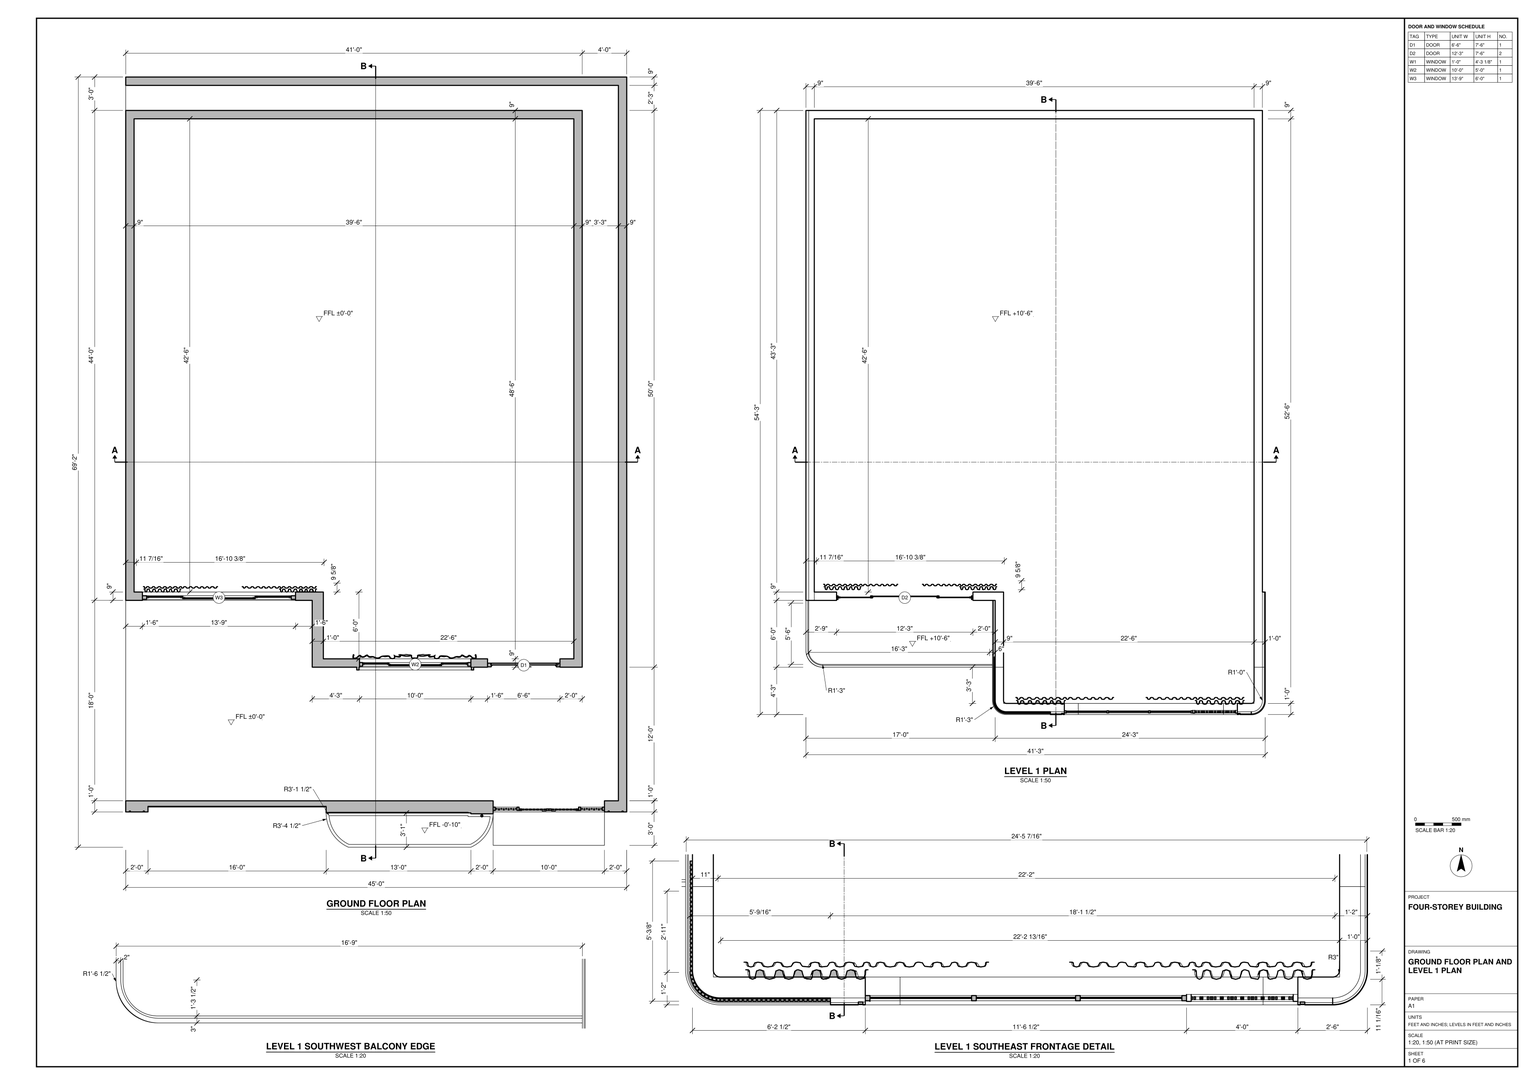
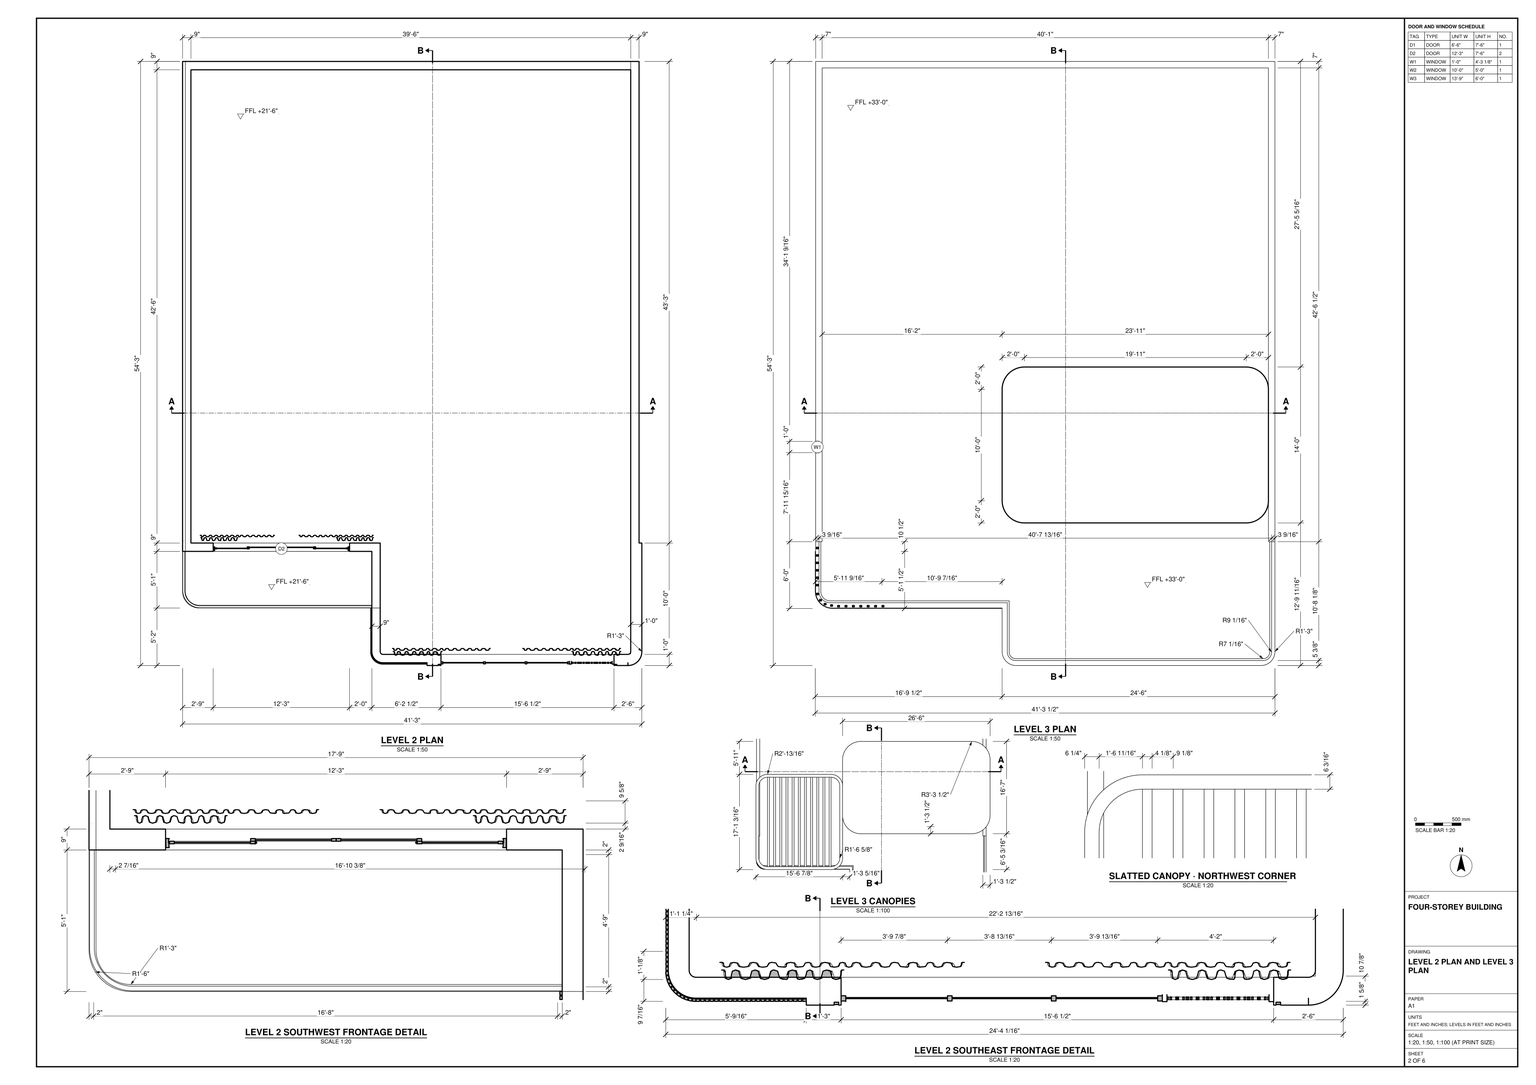
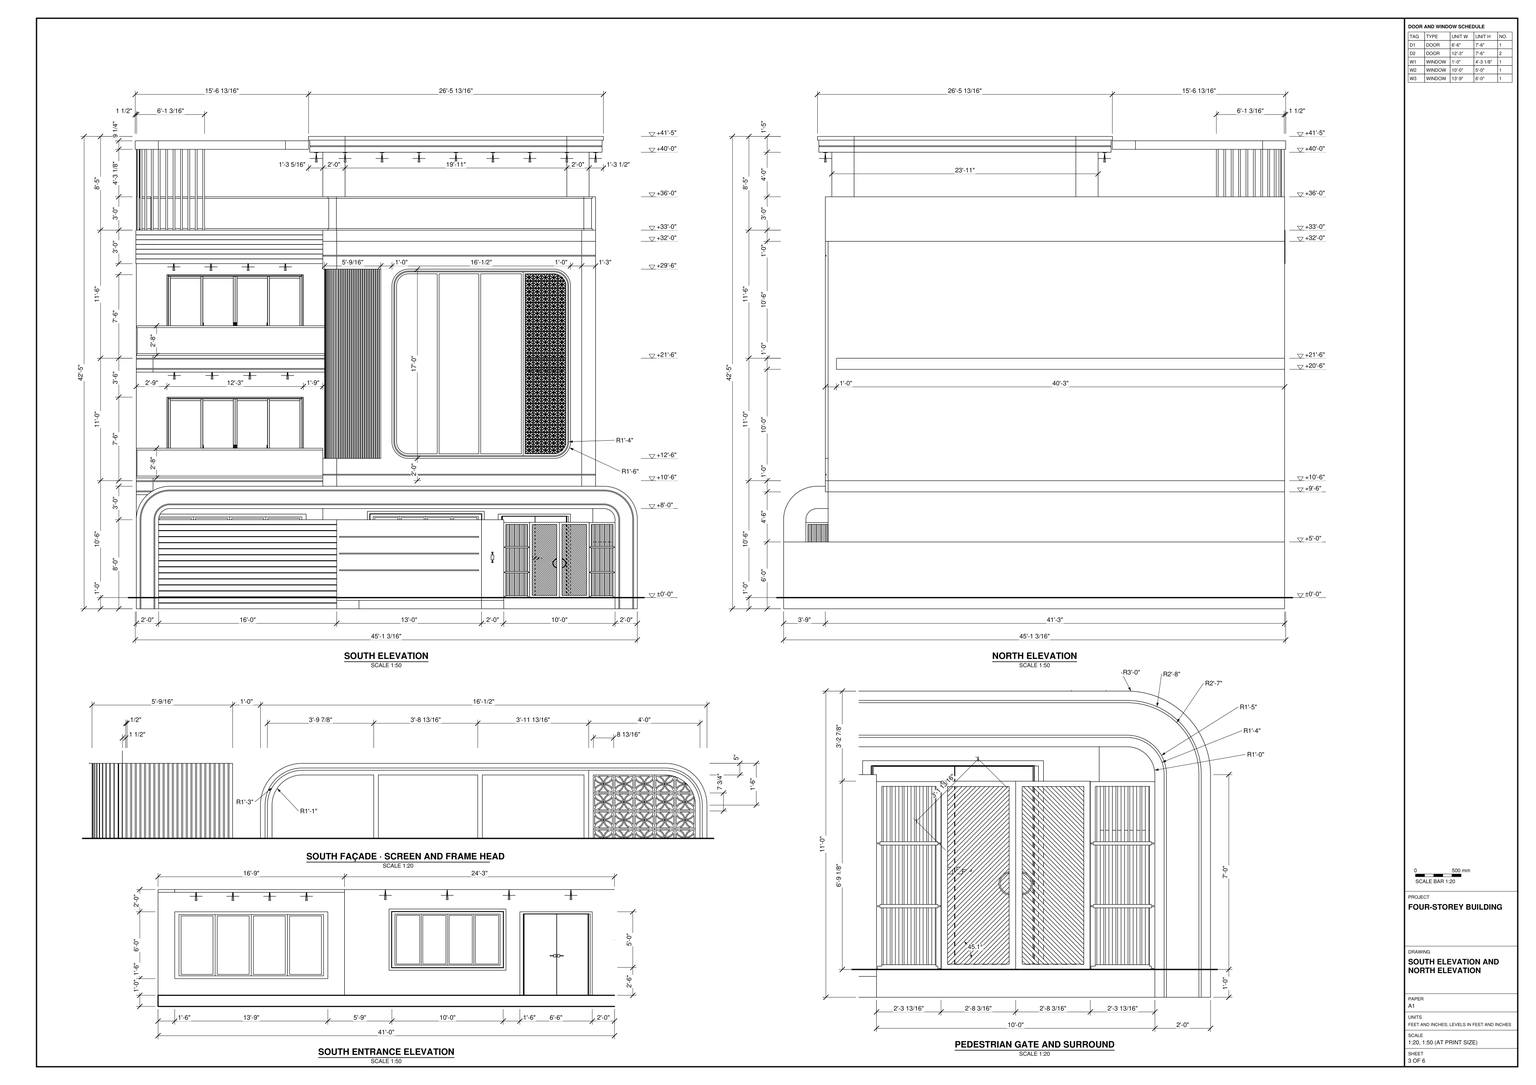
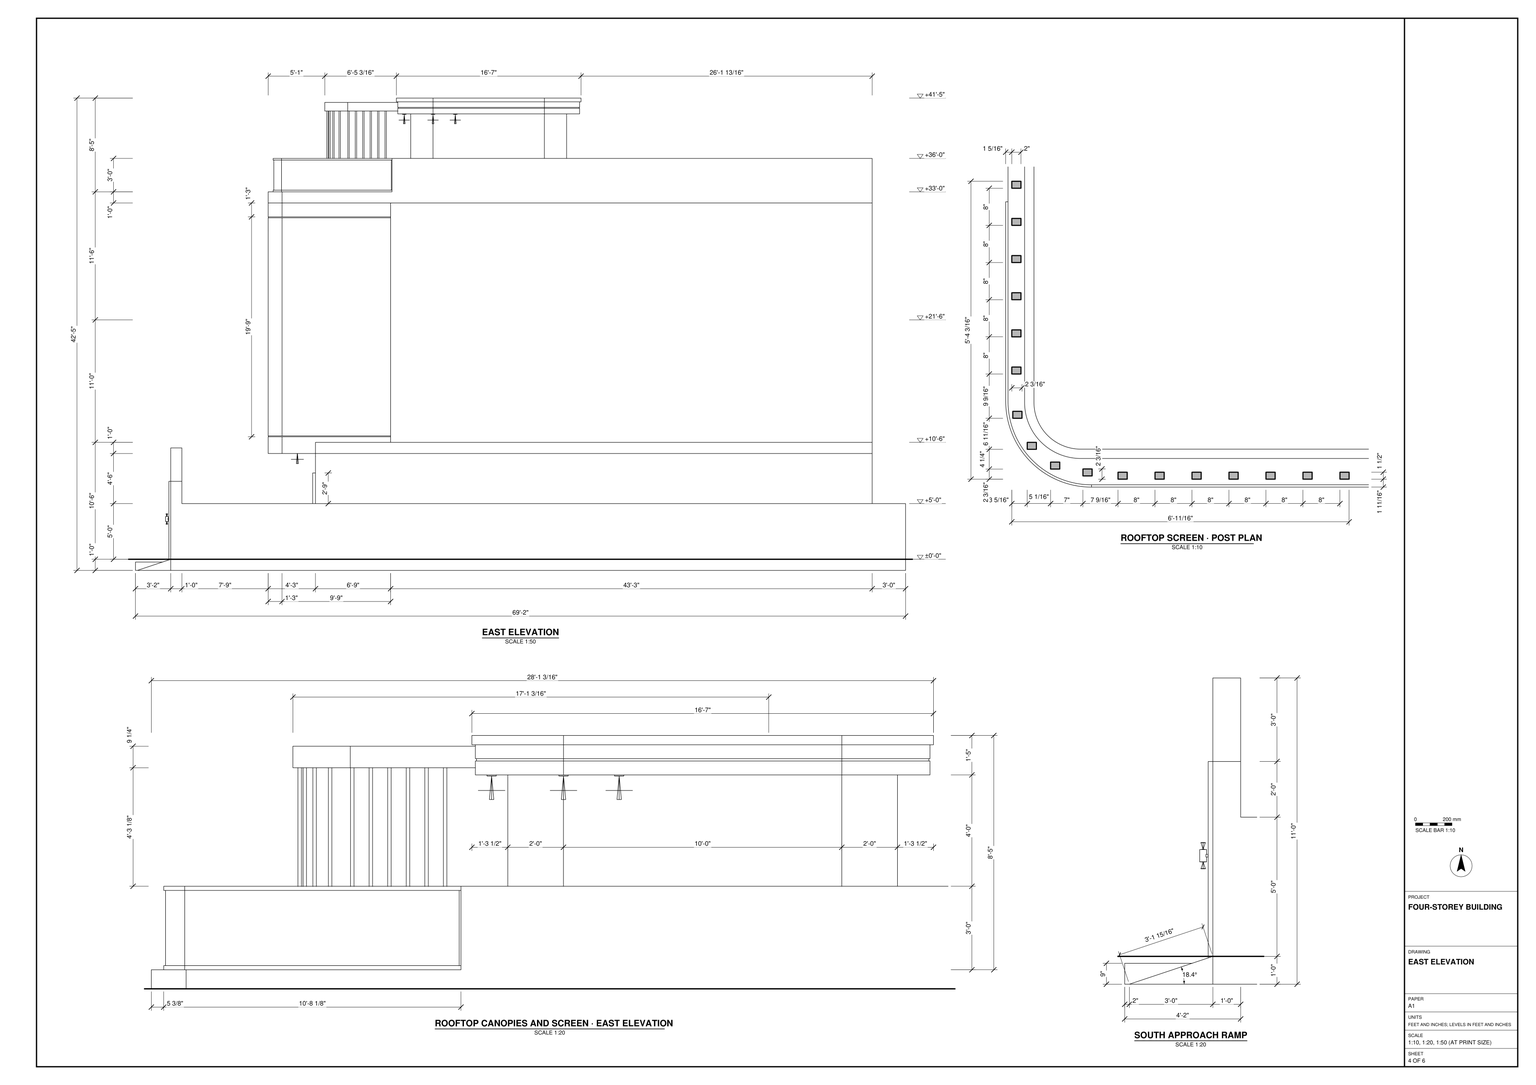
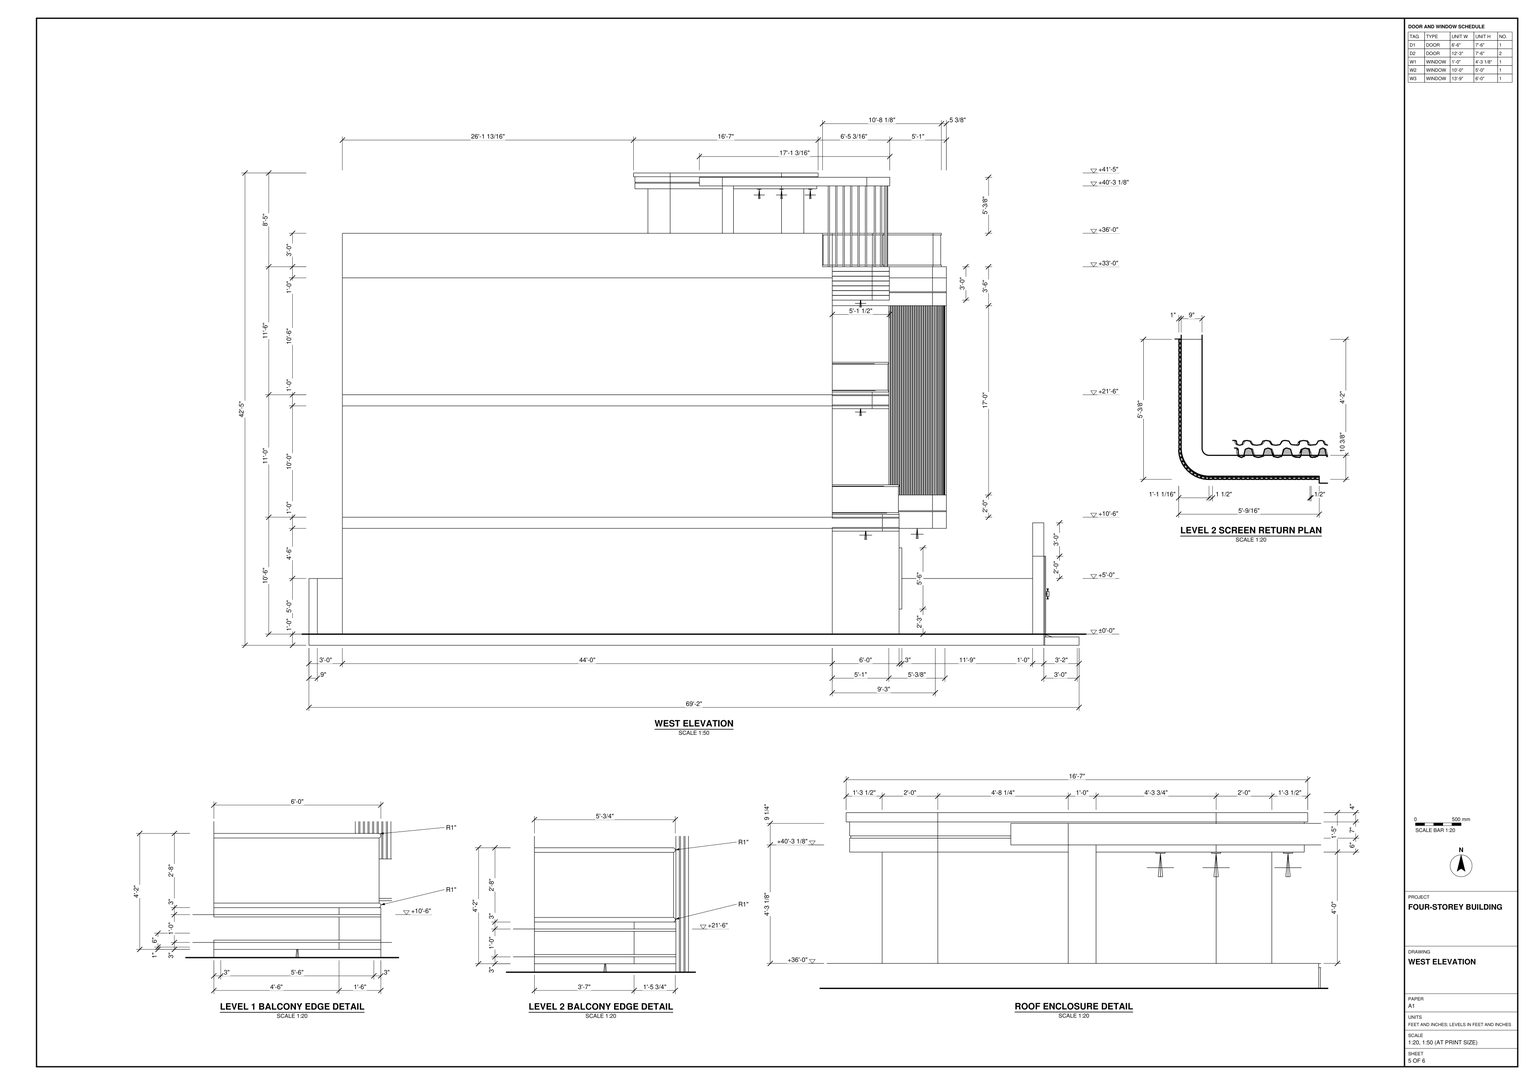
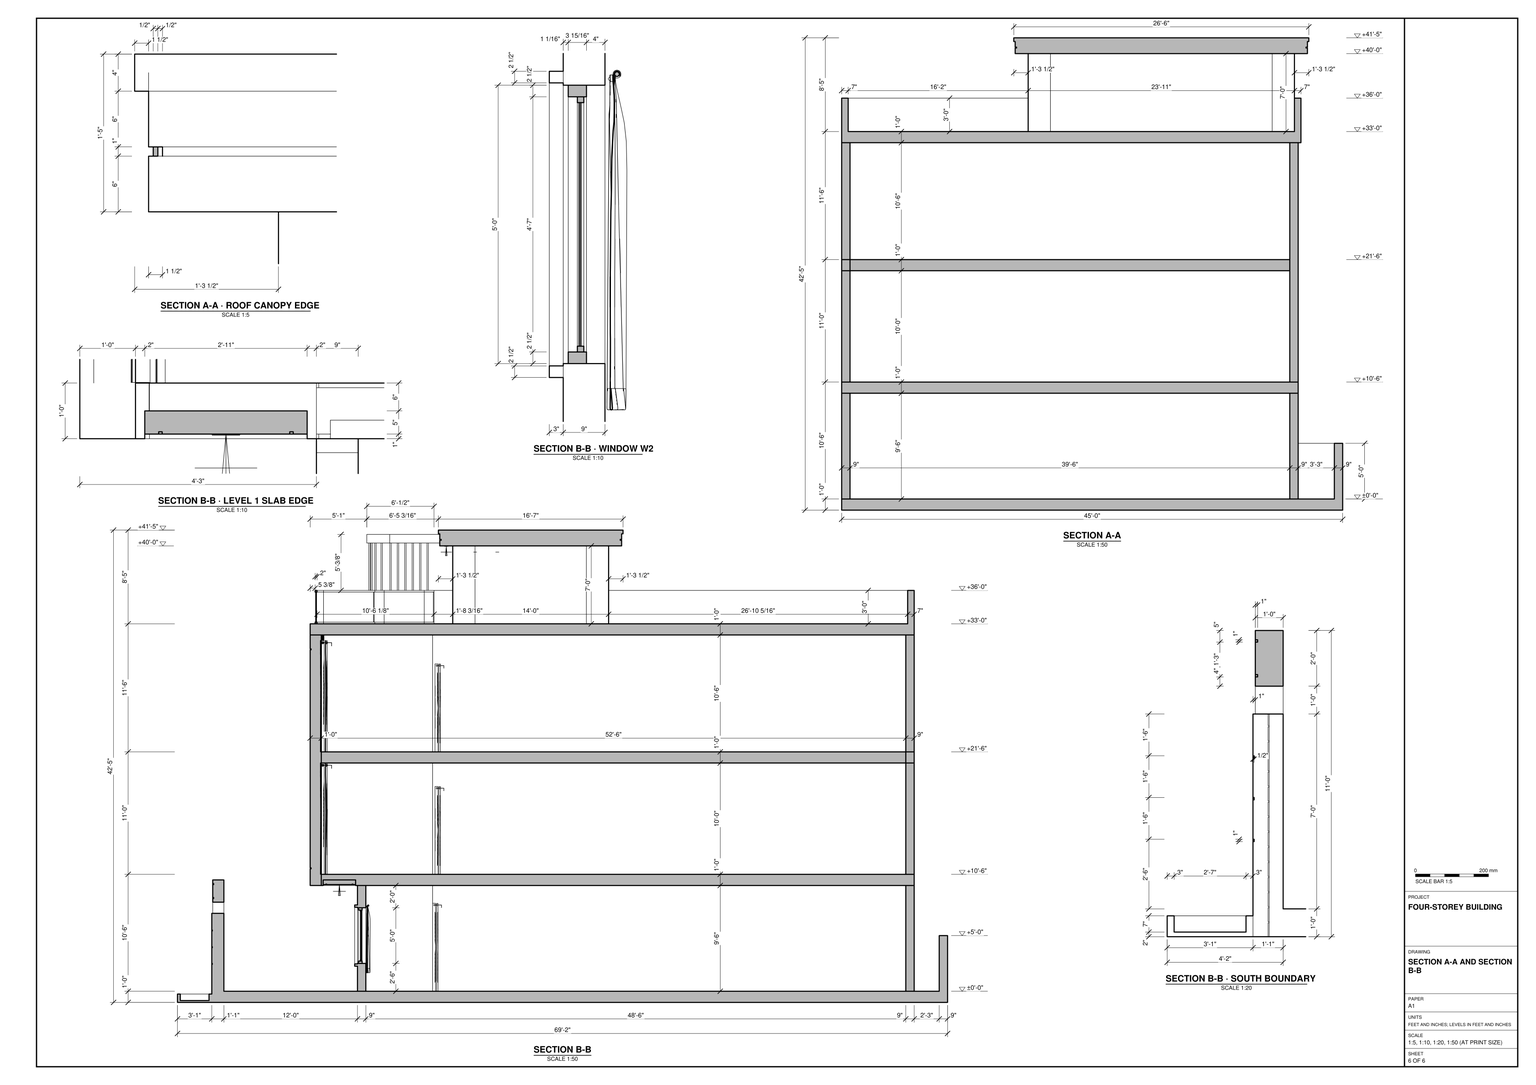
Use all six sheets in task_files/diagram_01.pdf to build the four-storey building in SketchUp. Work in feet and inches. The overall model, including the ground-level enclosure and rooftop canopies, is 45'-1 3/16" wide, 69'-2" deep and 42'-5" high. Set the ground floor at ±0'-0" and the successive floor levels at +10'-6", +21'-6" and +33'-0".

Lay out the perimeter enclosure and the building footprint separately so that the entrance façade sits behind the south gates. Model the floor slabs and walls with their thicknesses as drawn, including the steps in the south frontage. Fit the doors and windows to their scheduled openings. On the south elevation, distinguish the stacked southwest balconies from the projecting southeast bay. Model the balcony edges, the vertical fins and the tall rounded frame with its screened end panel. At ground level, include the rounded gate surround, the wide horizontal slats and the separate pedestrian gate. Finish the roof terrace with its parapet and the adjoining slatted and solid canopies. Include stairs, built-in joinery and main furniture where shown. Decor and loose items may be any suitable library components.

Keep shell elements such as walls, slabs and roof elements in separate groups or components. Group each furniture or joinery piece separately and use components for repeated parts. Save one SketchUp model as output_files/four_storey_building_with_stepped_balconies.skp.

# SketchUp Ruby script. Lengths in inches.
U = 1.inch
M = Sketchup.active_model
def pt(a) = Geom::Point3d.new(a.map { |v| v * U })
def face(e, loops, mat)
  f = e.add_face(loops[0].map { |a| pt(a) })
  loops[1..].each { |l| e.add_face(l.map { |a| pt(a) }).erase! }
  f.material = f.back_material = mat if mat
  f
end
# faces: each face lists its corners as indices into pts; further lists are holes
def faces(e, pts, list, mat = nil) = list.each { |f| face(e, (f[0].is_a?(Array) ? f : [f]).map { |l| l.map { |i| pts[i] } }, mat) }
# xy, xz, yz: faces in a plane at the given z, y or x. An outline is a flat list of corners, or four numbers for a rectangle; further outlines are holes
def ring(l) = l.size == 4 ? [[l[0], l[1]], [l[2], l[1]], [l[2], l[3]], [l[0], l[3]]] : l.each_slice(2).to_a
def flat(e, list, mat, &to3) = list.each { |f| face(e, (f[0].is_a?(Array) ? f : [f]).map { |l| ring(l).map { |u, v| to3.(u, v) } }, mat) }
def xy(e, z, list, mat = nil) = flat(e, list, mat) { |x, y| [x, y, z] }
def xz(e, y, list, mat = nil) = flat(e, list, mat) { |x, z| [x, y, z] }
def yz(e, x, list, mat = nil) = flat(e, list, mat) { |y, z| [x, y, z] }
def lines(e, pts, list) = list.each { |a, b| e.add_line(pt(pts[a]), pt(pts[b])) }
# prism: a flat outline (further loops are holes) pulled along v
def prism(e, loops, v, mat = nil)
  f = face(e, loops, mat); d = Geom::Vector3d.new(v.map { |x| x * U })
  f.pushpull(f.normal.samedirection?(d) ? d.length : -d.length)
end
def box(e, o, s, mat = nil) = prism(e, [[o, [o[0] + s[0], o[1], o[2]], [o[0] + s[0], o[1] + s[1], o[2]], [o[0], o[1] + s[1], o[2]]]], [0, 0, s[2]], mat)
def at(x, y, z, deg = 0) = Geom::Transformation.translation(pt([x, y, z])) * Geom::Transformation.rotation(ORIGIN, Z_AXIS, deg.degrees)
def axes(o, x, y, z) = Geom::Transformation.new([*x, 0, *y, 0, *z, 0, *pt(o).to_a, 1])
def part(name) = M.definitions.add(name)
# library, detail: a bought-in or finely detailed component or shape, given as its bounding box
def library(name, o, s) = part(name).tap { |d| box(d.entities, o, s) }
def detail(e, o, s) = box(e.add_group.entities, o, s)
def put(e, d, t, mat = nil) = e.add_instance(d, t).tap { |i| i.material = mat if mat }
def group(e, t, mat = nil) = e.add_group.tap { |g| g.transformation = t; g.material = mat if mat }.entities
root = M.entities
M.materials.add("T METAL").color = [42, 41, 39]
M.materials.add("[Color_B21]").color = [51, 12, 0]
M.materials.add("[Color_L25]").color = [117, 101, 92]
M.materials.add("[Quartz Light Brown]").color = [215, 212, 212]
M.materials.add("[Translucent_Glass_Gray]").color = [128, 128, 128]
M.materials.add("[Wood Veneer 01]").color = [93, 57, 34]
M.materials.add("[Wood Veneer 01]1").color = [120, 70, 37]
c1 = library("Garniza_zaclona",[1.52,0,0],[127.96,8.15,78.72])
c2 = library("WALL LIGHT 69",[4.19,4.05,-9.07],[4.61,5.7,17.71])
c3 = part("Window frame")
prism(c3.entities,[[[0,70.87,0],[0,0,0],[0,0,47.24],[0,70.87,47.24]],[[0,1.97,1.97],[0,68.9,1.97],[0,68.9,45.28],[0,1.97,45.28]]],[7.875,0,0])
c4 = part("Window sash")
xy(c4.entities,0,[[0,0,3.9375,16.73]])
xy(c4.entities,0.98,[[0,0.98,1.77,15.75],[1.77,0.98,2.85,15.75],[2.85,0.98,3.9375,15.75]])
xy(c4.entities,42.32,[[0,0.98,1.77,15.75],[1.77,0.98,2.85,15.75],[2.85,0.98,3.9375,15.75]])
xy(c4.entities,43.31,[[0,0,3.9375,16.73]])
xz(c4.entities,0,[[0,0,3.9375,43.31]])
xz(c4.entities,0.98,[[0,0.98,1.77,42.32],[1.77,0.98,2.85,42.32],[2.85,0.98,3.9375,42.32]])
xz(c4.entities,15.75,[[0,0.98,1.77,42.32],[1.77,0.98,2.85,42.32],[2.85,0.98,3.9375,42.32]])
xz(c4.entities,16.73,[[0,0,3.9375,43.31]])
yz(c4.entities,0,[[[0,0,16.73,43.31],[0.98,0.98,15.75,42.32]]])
yz(c4.entities,1.77,[[0.98,0.98,15.75,42.32]],"[Translucent_Glass_Gray]")
yz(c4.entities,2.85,[[0.98,0.98,15.75,42.32]],"[Translucent_Glass_Gray]")
yz(c4.entities,3.9375,[[[0,0,16.73,43.31],[0.98,0.98,15.75,42.32]]])
c5 = part("simple+window")
p = [[0,68.9,1.97],[0,35.43,1.97]]
lines(c5.entities,p,[[0,1]])
put(c5.entities,c3,at(0,0,0))
put(c5.entities,c4,axes([1.14,52.17,1.97],[0.71,0,0],[0,1,0],[0,0,1]))
put(c5.entities,c4,axes([1.14,1.97,1.97],[0.71,0,0],[0,1,0],[0,0,1]))
put(c5.entities,c4,axes([3.9375,18.7,1.97],[0.71,0,0],[0,1,0],[0,0,1]))
put(c5.entities,c4,axes([3.9375,35.43,1.97],[0.71,0,0],[0,1,0],[0,0,1]))
c6 = part("Door frame")
xy(c6.entities,0,[[0,0,0,3.9375,1.97,3.9375,1.97,1.97,2.36,1.97,2.36,1.18,2.17,1.18,2.17,0.85,1.97,0.85,1.97,0],[37.73,0,37.73,0.85,37.53,0.85,37.53,1.18,37.34,1.18,37.34,1.97,37.73,1.97,37.73,3.9375,39.7,3.9375,39.7,0]])
xy(c6.entities,82.45,[[2.36,1.18,37.34,1.97]])
xy(c6.entities,82.64,[[2.17,0.85,37.53,1.18]])
xy(c6.entities,82.84,[[1.97,0,37.73,0.85],[1.97,1.97,37.73,3.9375]])
xy(c6.entities,84.81,[[0,0,39.7,3.9375]],"[Color_B21]")
xz(c6.entities,0,[[0,0,1.97,0,1.97,82.84,37.73,82.84,37.73,0,39.7,0,39.7,84.81,0,84.81]],"[Color_L25]")
xz(c6.entities,0.85,[[1.97,0,2.17,0,2.17,82.64,37.53,82.64,37.53,0,37.73,0,37.73,82.84,1.97,82.84]],"[Color_L25]")
xz(c6.entities,1.18,[[2.17,0,2.36,0,2.36,82.45,37.34,82.45,37.34,0,37.53,0,37.53,82.64,2.17,82.64]],"[Color_B21]")
xz(c6.entities,1.97,[[1.97,0,1.97,82.84,37.73,82.84,37.73,0,37.34,0,37.34,82.45,2.36,82.45,2.36,0]])
xz(c6.entities,3.9375,[[0,0,0,84.81,39.7,84.81,39.7,0,37.73,0,37.73,82.84,1.97,82.84,1.97,0]],"[Color_B21]")
yz(c6.entities,0,[[0,0,3.9375,84.81]],"[Color_B21]")
yz(c6.entities,1.97,[[1.97,0,3.9375,82.84]])
yz(c6.entities,1.97,[[0,0,0.85,82.84]],"[Color_L25]")
yz(c6.entities,2.17,[[0.85,0,1.18,82.64]],"[Color_L25]")
yz(c6.entities,2.36,[[1.18,0,1.97,82.45]],"[Color_B21]")
yz(c6.entities,37.34,[[1.18,0,1.97,82.45]],"[Color_B21]")
yz(c6.entities,37.53,[[0.85,0,1.18,82.64]],"[Color_L25]")
yz(c6.entities,37.73,[[1.97,0,3.9375,82.84]])
yz(c6.entities,37.73,[[0,0,0.85,82.84]],"[Color_L25]")
yz(c6.entities,39.7,[[0,0,3.9375,84.81]],"[Color_B21]")
# 3 loose lines left out
c7 = part("Group\#13")
xy(c7.entities,0,[[0,2.36,35.76,4.33]])
xy(c7.entities,38.8,[[1.3,0,1.36,2.36],[1.36,0,3.29,2.36]],"[Color_L25]")
xy(c7.entities,39.63,[[3.29,0.09,3.54,0.79]],"[Color_L25]")
xy(c7.entities,39.85,[[3.54,0.09,7.14,0.79]],"[Color_L25]")
xy(c7.entities,39.86,[[7.15,0.09,7.16,0.79]],"[Color_L25]")
xy(c7.entities,40.55,[[7.15,0.09,7.17,0.79]],"[Color_L25]")
xy(c7.entities,40.5625,[[3.53,0.09,7.11,0.79],[7.11,0.09,7.125,0.79]],"[Color_L25]")
xy(c7.entities,40.8125,[[3.29,0.09,3.53,0.79]],"[Color_L25]")
xy(c7.entities,41.55,[[1.35,0,1.41,2.36],[1.41,0,3.29,2.36]],"[Color_L25]")
xy(c7.entities,82.84,[[0,2.36,35.76,4.33]])
xz(c7.entities,0,[[1.3,38.8,3.29,38.8,3.29,41.55,1.35,41.55,1.28,41.54,1.23,41.52,1.17,41.49,1.07,41.41,1.03,41.37,0.99,41.31,0.97,41.26,0.95,41.2,0.93,41.08,0.93,39.17,0.95,39.11,0.96,39.0625,0.99,39.01,1.02,38.96,1.06,38.92,1.1,38.89,1.14,38.85,1.19,38.83,1.25,38.8125]],"[Color_L25]")
xz(c7.entities,0.09,[[3.29,39.63,3.54,39.63,3.54,39.85,7.14,39.85,7.15,39.86,7.16,39.86,7.18,39.87,7.1875,39.875,7.2,39.88,7.21,39.89,7.22,39.91,7.22,39.92,7.23,39.93,7.23,40.47,7.22,40.49,7.2,40.51,7.19,40.53,7.17,40.55,7.15,40.55,7.14,40.56,7.125,40.5625,3.53,40.5625,3.53,40.8125,3.29,40.8125]],"[Color_L25]")
xz(c7.entities,0.79,[[3.29,39.63,3.29,40.8125,3.53,40.8125,3.53,40.5625,7.125,40.5625,7.14,40.56,7.15,40.55,7.17,40.55,7.19,40.53,7.2,40.51,7.22,40.49,7.23,40.47,7.23,39.93,7.22,39.92,7.22,39.91,7.21,39.89,7.2,39.88,7.1875,39.875,7.18,39.87,7.16,39.86,7.15,39.86,7.14,39.85,3.54,39.85,3.54,39.63]],"[Color_L25]")
xz(c7.entities,2.36,[[[0,0,35.76,82.84],[0.93,38.8,3.29,41.55]],[0.93,38.8,1.36,38.8,1.3,38.8,1.25,38.8125,1.19,38.83,1.14,38.85,1.1,38.89,1.06,38.92,1.02,38.96,0.99,39.01,0.96,39.0625,0.95,39.11,0.93,39.17,0.93,39.22],[0.93,41.08,0.95,41.2,0.97,41.26,0.99,41.31,1.03,41.37,1.07,41.41,1.17,41.49,1.23,41.52,1.28,41.54,1.35,41.55,1.41,41.55,0.93,41.55]],"[Color_L25]")
xz(c7.entities,4.33,[[0,0,35.76,82.84]])
yz(c7.entities,0,[[2.36,0,4.33,82.84]])
yz(c7.entities,0.93,[[0,39.17,2.36,39.22],[0,39.22,2.36,41.08]],"[Color_L25]")
yz(c7.entities,3.29,[[[0,38.8,2.36,41.55],[0.09,39.63,0.79,40.8125]]],"[Color_L25]")
yz(c7.entities,3.53,[[0.09,40.5625,0.79,40.8125]],"[Color_L25]")
yz(c7.entities,3.54,[[0.09,39.63,0.79,39.85]],"[Color_L25]")
yz(c7.entities,7.22,[[0.09,39.91,0.79,39.92]],"[Color_L25]")
yz(c7.entities,7.23,[[0.09,39.93,0.79,39.94],[0.09,39.94,0.79,40.4375],[0.09,40.4375,0.79,40.46],[0.09,40.46,0.79,40.47]],"[Color_L25]")
yz(c7.entities,35.76,[[2.36,0,4.33,82.84]])
# 3 loose lines left out
p = [[1.19,0,38.83],[1.14,0,38.85],[1.14,2.36,38.85],[1.19,2.36,38.83],[1.3,0,38.8],[1.25,0,38.8125],
  [1.25,2.36,38.8125],[1.3,2.36,38.8],[1.06,0,38.92],[1.02,0,38.96],[1.02,2.36,38.96],[1.06,2.36,38.92],
  [1.1,0,38.89],[1.1,2.36,38.89],[0.99,0,39.01],[0.99,2.36,39.01],[0.96,0,39.0625],[0.96,2.36,39.0625],
  [0.95,0,39.11],[0.95,2.36,39.11],[0.93,0,39.17],[0.93,2.36,39.17],[7.15,0.09,39.86],[7.14,0.09,39.85],
  [7.14,0.79,39.85],[7.15,0.79,39.86],[7.22,0.09,39.91],[7.21,0.09,39.89],[7.21,0.79,39.89],[7.22,0.79,39.91],
  [7.2,0.09,39.88],[7.2,0.79,39.88],[7.1875,0.09,39.875],[7.1875,0.79,39.875],[7.18,0.09,39.87],[7.18,0.79,39.87],
  [7.16,0.09,39.86],[7.16,0.79,39.86],[7.23,0.09,39.93],[7.22,0.09,39.92],[7.22,0.79,39.92],[7.23,0.79,39.93],
  [7.17,0.09,40.55],[7.18,0.09,40.54],[7.18,0.79,40.54],[7.17,0.79,40.55],[7.19,0.09,40.53],[7.19,0.79,40.53],
  [7.2,0.09,40.51],[7.2,0.79,40.51],[7.21,0.09,40.5],[7.21,0.79,40.5],[7.22,0.09,40.49],[7.22,0.79,40.49],
  [7.23,0.09,40.47],[7.23,0.79,40.47],[7.125,0.09,40.5625],[7.14,0.09,40.56],[7.14,0.79,40.56],[7.125,0.79,40.5625],
  [7.15,0.09,40.55],[7.15,0.79,40.55],[0.93,0,41.08],[0.94,0,41.14],[0.94,2.36,41.14],[0.93,2.36,41.08],
  [0.95,0,41.2],[0.95,2.36,41.2],[0.97,0,41.26],[0.97,2.36,41.26],[0.99,0,41.31],[0.99,2.36,41.31],
  [1.03,0,41.37],[1.03,2.36,41.37],[1.07,0,41.41],[1.07,2.36,41.41],[1.12,0,41.45],[1.12,2.36,41.45],
  [1.17,0,41.49],[1.17,2.36,41.49],[1.23,0,41.52],[1.23,2.36,41.52],[1.28,0,41.54],[1.28,2.36,41.54],
  [1.35,0,41.55],[1.35,2.36,41.55]]
faces(c7.entities,p,[[0,1,2,3],[4,5,6,7],[5,0,3,6],[8,9,10,11],[1,12,13,2],[12,8,11,13],[9,14,15,10],[14,16,17,15],
  [16,18,19,17],[18,20,21,19],[22,23,24,25],[26,27,28,29],[27,30,31,28],[30,32,33,31],[32,34,35,33],[34,36,37,35],
  [38,39,40,41],[42,43,44,45],[43,46,47,44],[46,48,49,47],[48,50,51,49],[50,52,53,51],[52,54,55,53],[56,57,58,59],
  [57,60,61,58],[62,63,64,65],[63,66,67,64],[66,68,69,67],[68,70,71,69],[70,72,73,71],[72,74,75,73],[74,76,77,75],
  [76,78,79,77],[78,80,81,79],[80,82,83,81],[82,84,85,83]],"[Color_L25]")
c8 = part("Elegant door(double)")
p = [[77.86,31.43,0],[42.82,31.43,0],[38.88,31.43,0]]
lines(c8.entities,p,[[0,1],[1,2]])
put(c8.entities,c6,axes([38.88,29.47,0],[1.93222,0,0],[0,1,0],[0,0,1]),"[Color_B21]")
put(c8.entities,c7,at(77.86,29.07,0),"[Wood Veneer 01]1")
put(c8.entities,c7,axes([78.05,29.07,0],[-1,0,0],[0,1,0],[0,0,1]),"[Wood Veneer 01]1")
c9 = library("SHOWER+CURTAIN",[-76.11,-2.58,2.78],[135.11,4.99,73.24])
c10 = library("Group\#16",[0,-39,-17.9],[492,639,58.9])
c11 = library("Group\#2",[0,-51,-12],[495,651,276])
c12 = library("Group\#17",[-9,0,-16.51],[483,639,57.51])
c13 = library("Group\#41",[0,-194,-12],[540,830,132])
c14 = library("Group\#44",[-0.5,0,-31.51],[495.5,651,79.51])
c15 = library("Group\#50",[0,0,0],[287,168,84])
c16 = library("Group\#51",[-15.5,-15.5,-10.61],[318,199,27.61])
c17 = library("Group\#53",[0,0,-93.56],[180,199,93.56])
put(root,c1,axes([213,-36.96,126],[2.08532,0,0],[0,1.49,0],[0,0,1.52445]))
put(root,c1,axes([213,-36.96,258],[2.08532,0,0],[0,1.49,0],[0,0,1.52445]))
put(root,c1,axes([9,86.55,258],[1.58151,0,0],[0,1.1771,0],[0,0,1.20432]))
put(root,c1,axes([9,86.55,125.89],[1.58151,0,0],[0,1.1771,0],[0,0,1.20432]))
put(root,c2,axes([379.65,-161.24,43.54],[0.64,0,0],[0,0.64,0],[0,0,0.64]))
g1 = group(root,at(0,3,0),"[Quartz Light Brown]")
put(g1,c1,axes([9,81,0],[1.58151,0,0],[0,1.1771,0],[0,0,1.20432]))
g2 = group(g1,at(0,0,0))
xy(g2,0,[[201,0,201,72,0,72,0,600,492,600,492,0,468,0,468,9,483,9,483,591,9,591,9,81,213,81,213,9,390,9,390,0]])
xy(g2,18,[[18,72,183,81]])
xy(g2,27,[[249,-3,375,0]])
xy(g2,29.5,[[251.5,-3,372.5,0]])
xy(g2,30,[[252,0,372,9]])
xy(g2,90,[[252,0,372,9],[390,0,468,9],[18,72,183,81]])
xy(g2,90.5,[[251.5,-3,372.5,0]])
xy(g2,93,[[249,-3,375,0]])
xy(g2,114,[[[201,0,492,0,492,600,0,600,0,72,201,72],[213,9,213,81,9,81,9,591,483,591,483,9]]])
xz(g2,-3,[[[249,27,375,93],[251.5,29.5,372.5,90.5]]])
xz(g2,0,[[[201,0,390,0,390,90,468,90,468,0,492,0,492,114,201,114],[249,27,375,93]],[[251.5,29.5,372.5,90.5],[252,30,372,90]],[372.5,29.5,373,91.5],[373,29.5,373.5,91.5]])
xz(g2,9,[[[213,0,213,114,483,114,483,0,468,0,468,90,390,90,390,0],[252,30,372,90]]])
xz(g2,72,[[[0,0,201,114],[18,18,183,90]]])
xz(g2,81,[[[9,0,213,114],[18,18,183,90]]])
xz(g2,591,[[9,0,483,114]])
xz(g2,600,[[0,0,492,114]])
yz(g2,0,[[72,0,600,114]])
yz(g2,9,[[81,0,591,114]])
yz(g2,18,[[72,18,81,90]])
yz(g2,183,[[72,18,81,90]])
yz(g2,201,[[0,0,72,114]])
yz(g2,213,[[9,0,81,114]])
yz(g2,249,[[-3,27,0,93]])
yz(g2,251.5,[[-3,29.5,0,90.5]])
yz(g2,252,[[0,30,9,90]])
yz(g2,372,[[0,30,9,90]])
yz(g2,372.5,[[-3,29.5,0,90.5]])
yz(g2,375,[[-3,27,0,93]])
yz(g2,390,[[0,0,9,90]])
yz(g2,468,[[0,0,9,90]])
yz(g2,483,[[9,0,591,114]])
yz(g2,492,[[0,0,600,114]])
put(g2,c5,axes([252,5.01,30],[0,-0.5,0],[1.69333,0,0],[0,0,1.27]),"T METAL")
put(g2,c8,axes([350.47,-29.07,0],[1.01686,0,0],[0,1,0],[0,0,1.0612]))
put(g2,c5,axes([18,77.01,18],[0,-0.5,0],[2.32833,0,0],[0,0,1.524]),"T METAL")
put(g2,c9,at(319.92,11.58,17.23))
put(g1,c10,at(0,0,120))
put(g1,c11,at(0,0,126))
put(g1,c12,at(9,-39,252))
put(g1,c13,at(0,0,0))
put(g1,c14,at(0,-51,384))
put(g1,c15,at(201,102.68,396))
put(g1,c16,at(201,102.7,480))
put(g1,c17,axes([-1.1875,10.03,492.37],[1.03803,0,0],[0,1.03103,0],[0,0,1.03]),"[Wood Veneer 01]")
